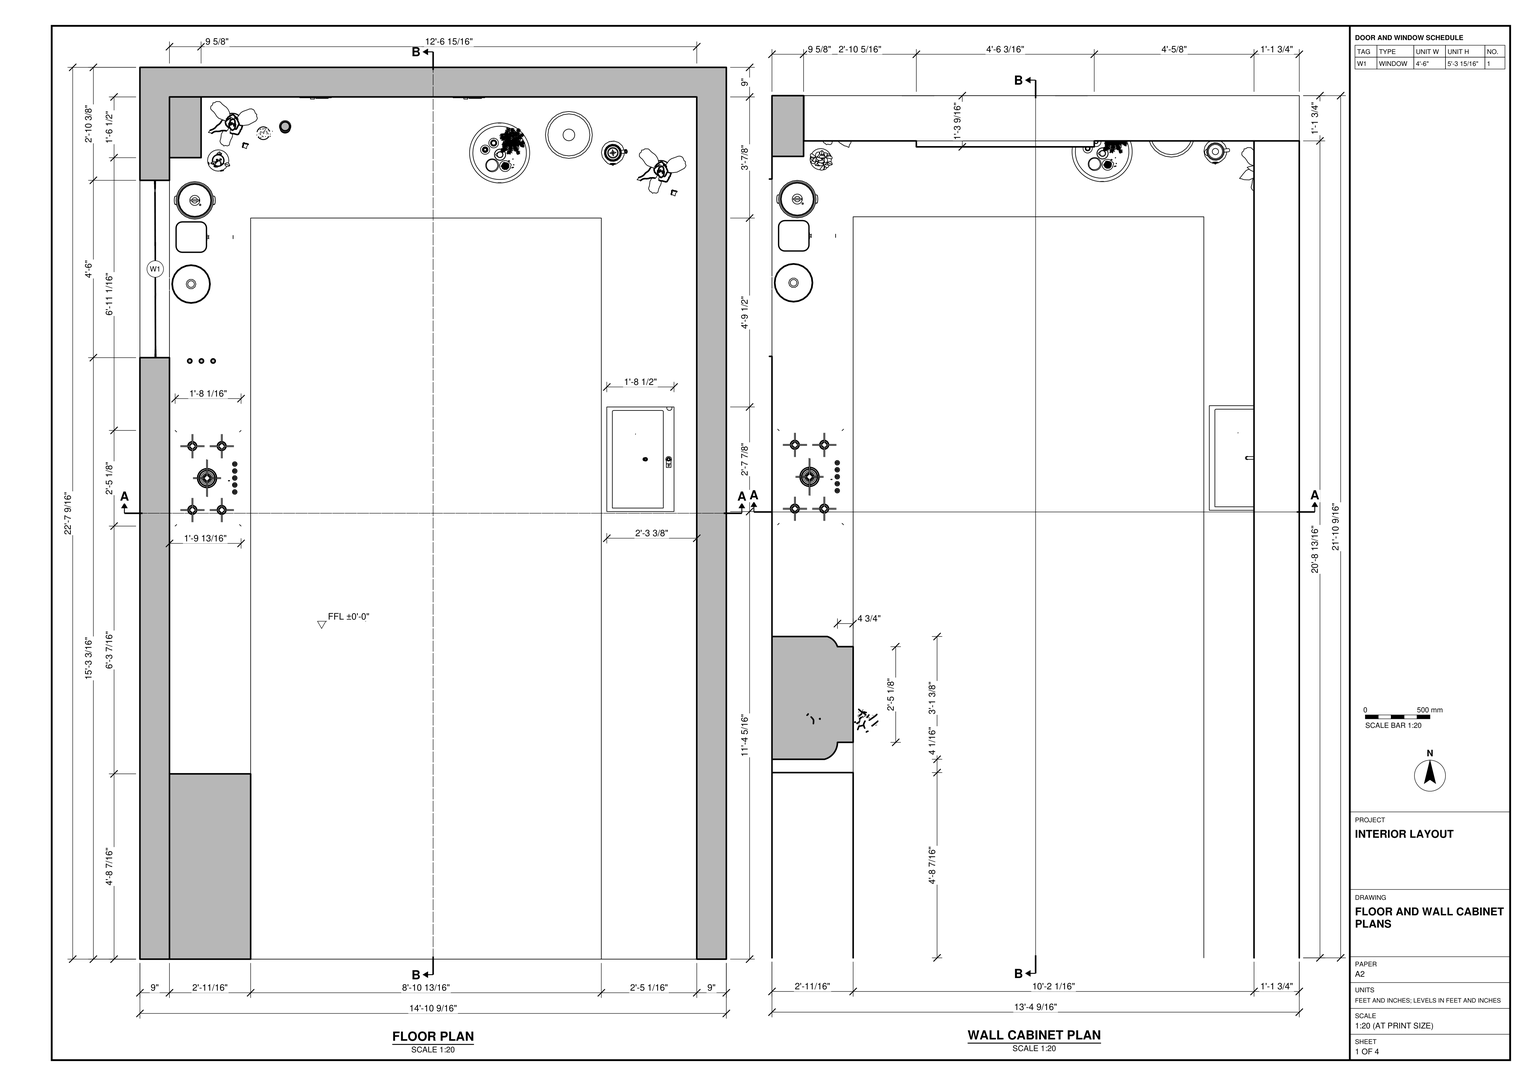
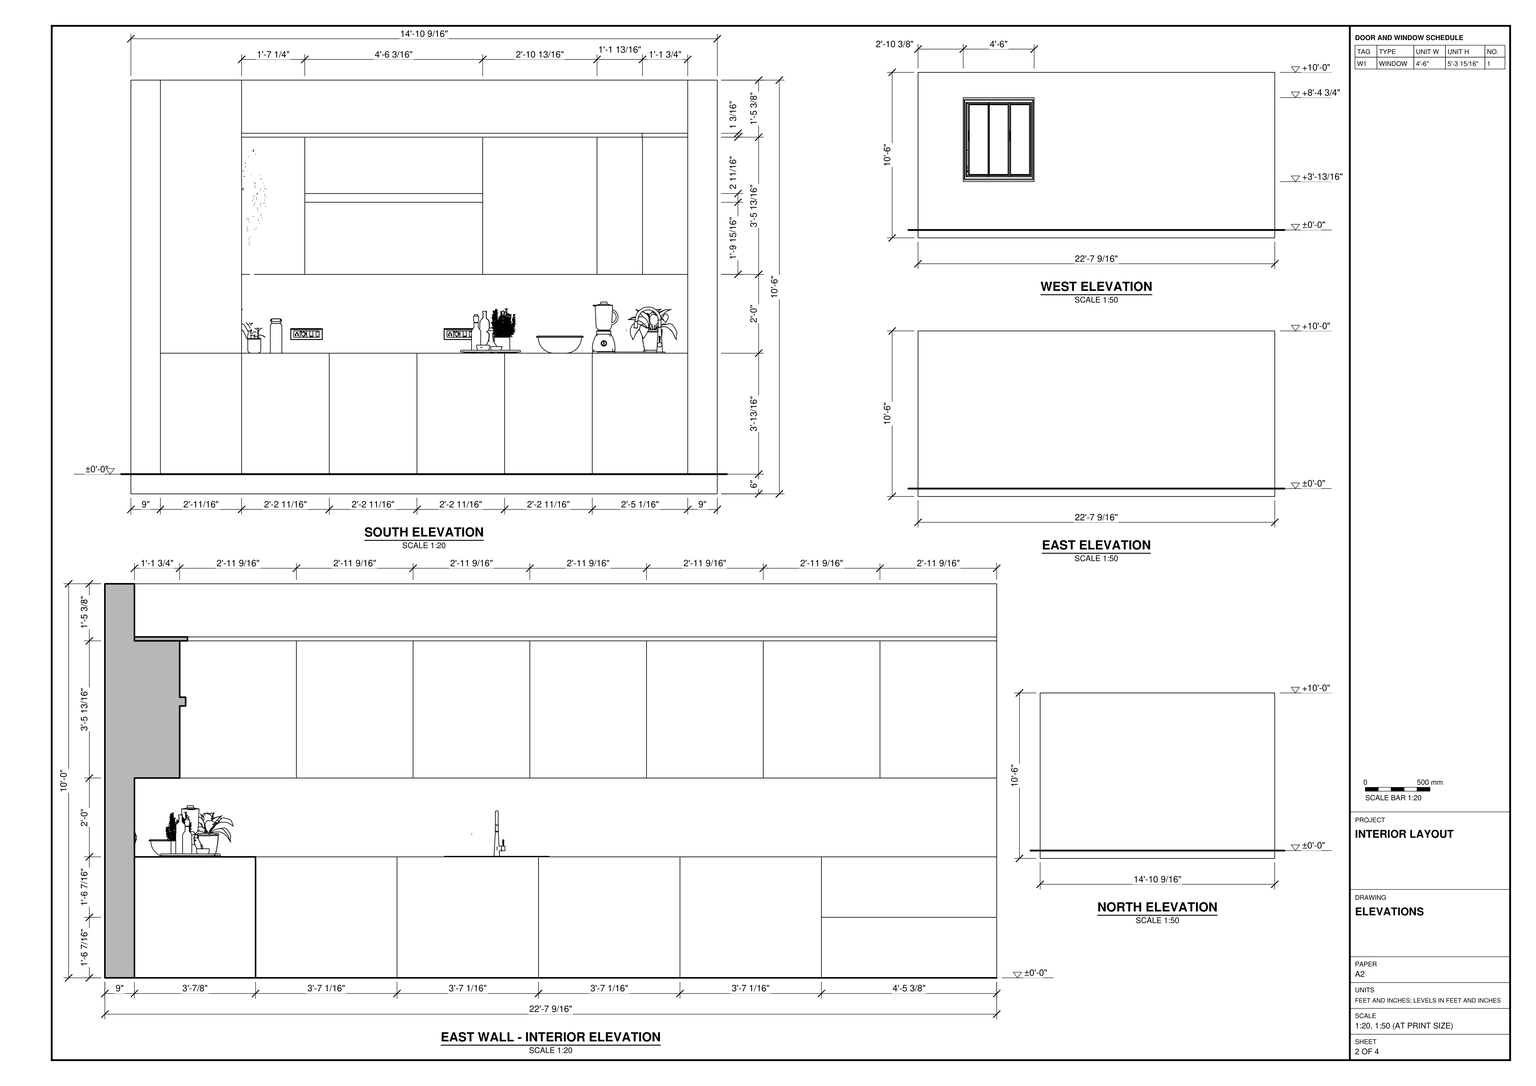
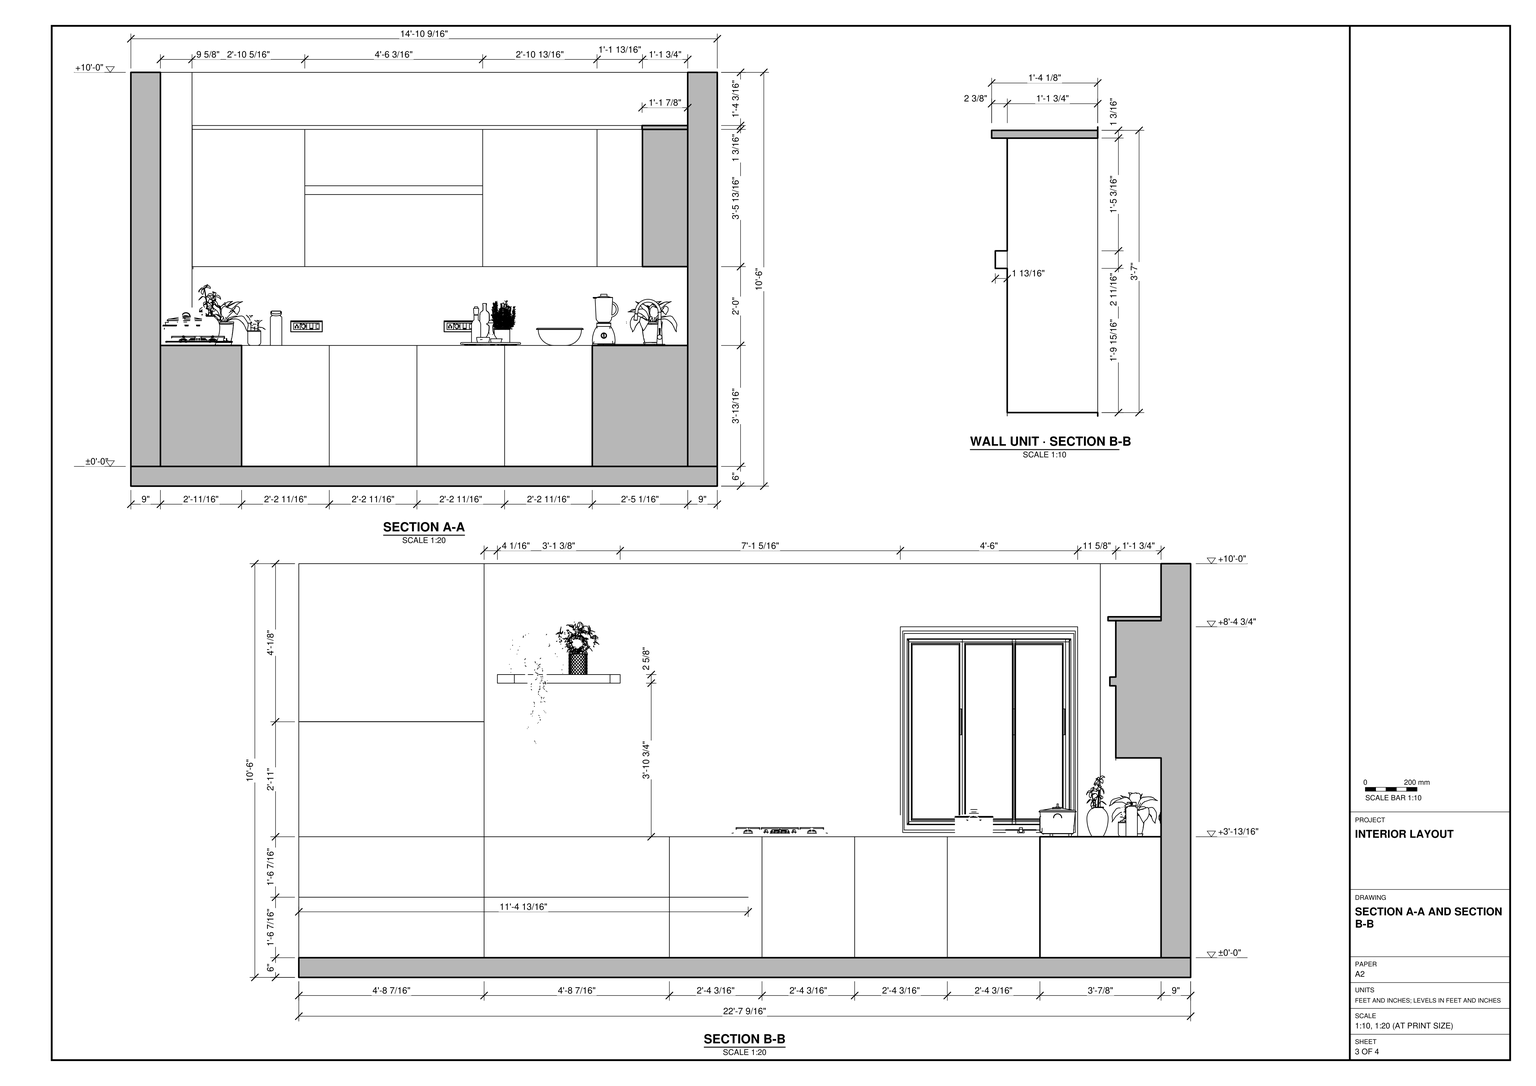
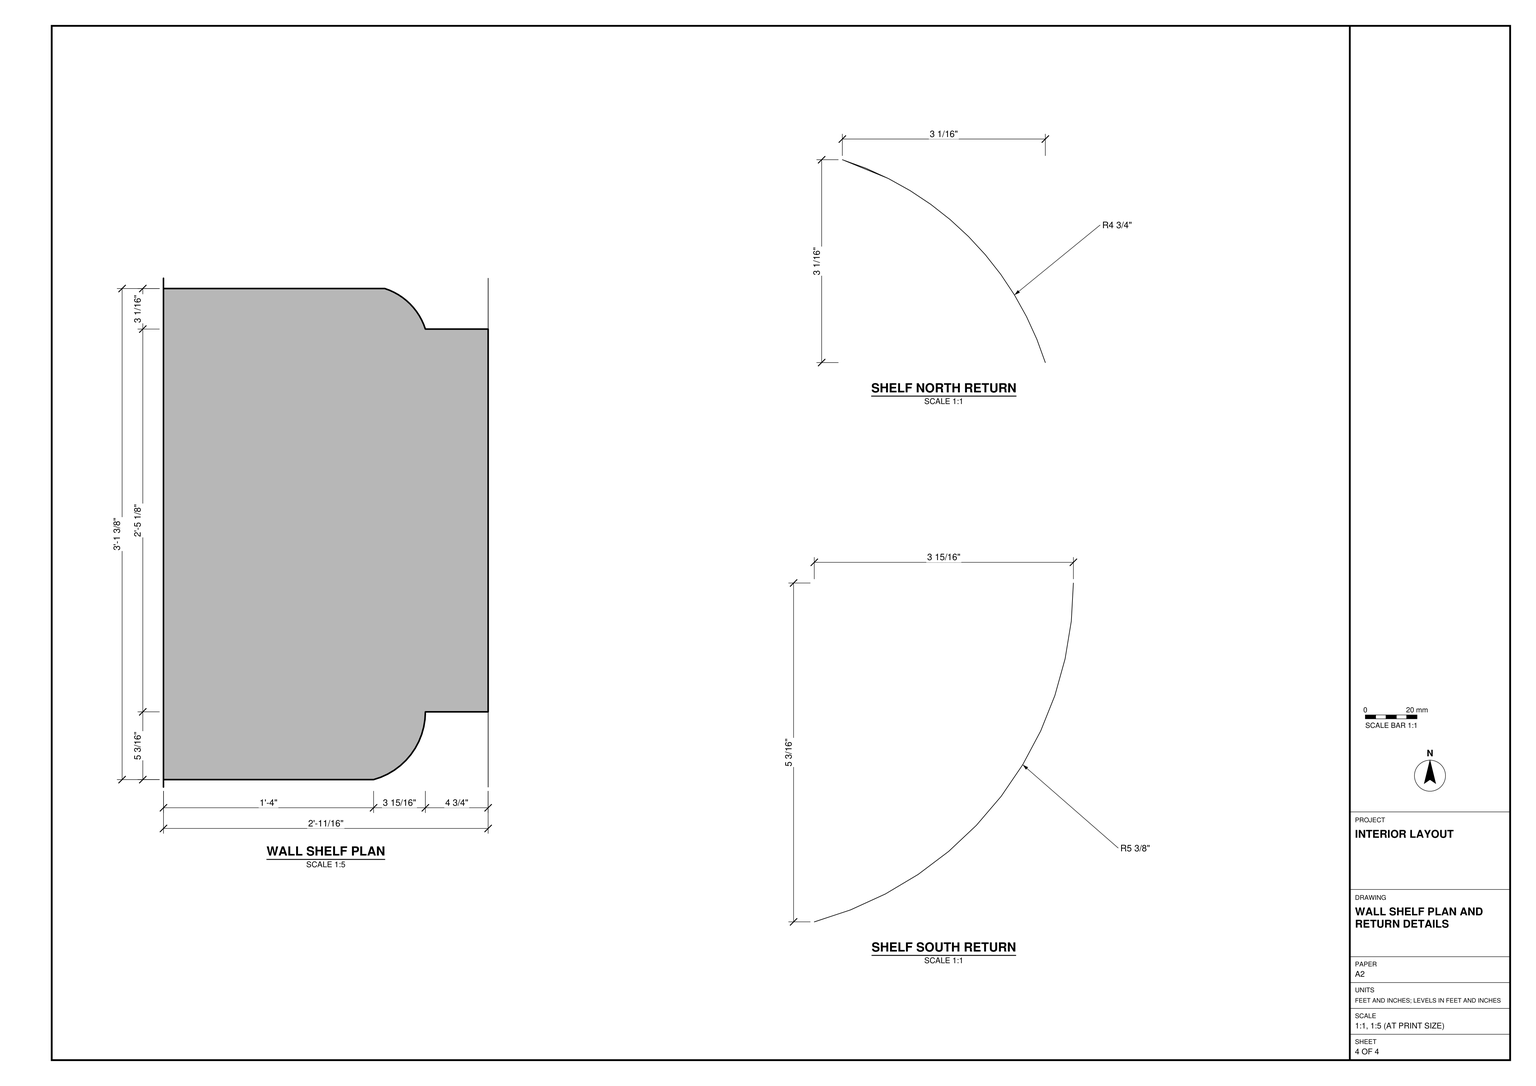
Build the kitchen interior in SketchUp from task_files/diagram_01.pdf. Work in feet and inches. Set the finished floor at ±0'-0". The overall model is 14'-10 9/16" wide, 22'-7 9/16" long and 10'-6" high, including the 6" floor slab below the finished floor. Build the 9" walls on the west, north and east sides, leaving the south end open. Fit the framed window into the west wall at the location and sill height shown.

Run the base cabinets and worktops along both sides and across the north end, keeping the central aisle clear. Place the cooktop on the west run and the sink and tap opposite it on the east run. Use the elevations and sections to set out the cabinet fronts, the tall unit at the open end of the west run and the wall shelf beside it. Model the wall cabinets along the north and east walls, matching their bay widths, projecting top trim and clearance above the worktop. Decor and loose items, including plants, kitchenware and countertop appliances, may be any suitable library components placed as shown.

Keep the shell elements and each piece of joinery or furniture in separate groups or components, and use components for repeated parts. Save one SketchUp model as output_files/open_ended_kitchen_with_u_shaped_cabinetry.skp.

# SketchUp Ruby script. Lengths in inches.
U = 1.inch
M = Sketchup.active_model
def pt(a) = Geom::Point3d.new(a.map { |v| v * U })
def face(e, loops, mat)
  f = e.add_face(loops[0].map { |a| pt(a) })
  loops[1..].each { |l| e.add_face(l.map { |a| pt(a) }).erase! }
  f.material = f.back_material = mat if mat
  f
end
# faces: each face lists its corners as indices into pts; further lists are holes
def faces(e, pts, list, mat = nil) = list.each { |f| face(e, (f[0].is_a?(Array) ? f : [f]).map { |l| l.map { |i| pts[i] } }, mat) }
# xy, xz, yz: faces in a plane at the given z, y or x. An outline is a flat list of corners, or four numbers for a rectangle; further outlines are holes
def ring(l) = l.size == 4 ? [[l[0], l[1]], [l[2], l[1]], [l[2], l[3]], [l[0], l[3]]] : l.each_slice(2).to_a
def flat(e, list, mat, &to3) = list.each { |f| face(e, (f[0].is_a?(Array) ? f : [f]).map { |l| ring(l).map { |u, v| to3.(u, v) } }, mat) }
def xy(e, z, list, mat = nil) = flat(e, list, mat) { |x, y| [x, y, z] }
def xz(e, y, list, mat = nil) = flat(e, list, mat) { |x, z| [x, y, z] }
def yz(e, x, list, mat = nil) = flat(e, list, mat) { |y, z| [x, y, z] }
def lines(e, pts, list) = list.each { |a, b| e.add_line(pt(pts[a]), pt(pts[b])) }
# prism: a flat outline (further loops are holes) pulled along v
def prism(e, loops, v, mat = nil)
  f = face(e, loops, mat); d = Geom::Vector3d.new(v.map { |x| x * U })
  f.pushpull(f.normal.samedirection?(d) ? d.length : -d.length)
end
def box(e, o, s, mat = nil) = prism(e, [[o, [o[0] + s[0], o[1], o[2]], [o[0] + s[0], o[1] + s[1], o[2]], [o[0], o[1] + s[1], o[2]]]], [0, 0, s[2]], mat)
def at(x, y, z, deg = 0) = Geom::Transformation.translation(pt([x, y, z])) * Geom::Transformation.rotation(ORIGIN, Z_AXIS, deg.degrees)
def axes(o, x, y, z) = Geom::Transformation.new([*x, 0, *y, 0, *z, 0, *pt(o).to_a, 1])
def part(name) = M.definitions.add(name)
# library, detail: a bought-in or finely detailed component or shape, given as its bounding box
def library(name, o, s) = part(name).tap { |d| box(d.entities, o, s) }
def detail(e, o, s) = box(e.add_group.entities, o, s)
def put(e, d, t, mat = nil) = e.add_instance(d, t).tap { |i| i.material = mat if mat }
def group(e, t, mat = nil) = e.add_group.tap { |g| g.transformation = t; g.material = mat if mat }.entities
root = M.entities
M.materials.add("[Color M01]").color = [226, 226, 226]
M.materials.add("[Color M04]").color = [142, 142, 142]
M.materials.add("[Tile Border Travertine]").color = [160, 142, 112]
M.materials.add("[Wood Bamboo]").color = [177, 105, 43]
M.materials.add("[Wood Floor Light]").color = [204, 176, 127]
c1 = library("WINDOW",[0,-0.02,0],[73.51,8.29,49.21])
c2 = library("mixer+blender",[-3.57,-3.85,0],[8.2,7.51,15.59])
c3 = library("MixingBowl",[0.58,0.58,0],[14.29,14.29,5.25])
c4 = library("kitchen",[57.57,5.21,10.61],[18.31,18.31,13.72])
c5 = library("Kitchen Pot",[-7.65,-5.94,0],[15.3,11.88,8.57])
c6 = library("Kitchen Pan",[-4.76,-4.76,0],[17.5,9.52,2.79])
c7 = library("Small Plant for Nightstand",[-0.92,-1.74,0],[6.62,5.06,9.81])
c8 = library("Untitled (1)",[45.65,19.99,0],[14.9,14.7,13.43])
c9 = library("Wall switch panel",[0,0,0],[9.65,3.39,0.65])
c10 = library("rice pan",[-4.26,-4.59,0],[12.51,11.42,10.02])
c11 = library("Küche",[96.12,-390.13,36.84],[20.08,114.94,19.93])
c12 = library("sink",[-18.39,0,-25.75],[31.85,20.47,39.62])
c13 = library("water bottle",[-1.75,-2.08,0],[3.5,3.83,10.5])
c14 = library("Untitled\#2",[167.21,48.36,-0.87],[34.16,22.4,50.98])
c15 = library("ARRANJO+ROSAS+BRANCAS",[219.65,-5.05,84.62],[22.21,22.69,31.57])
xy(root,102.625,[[155.67,0,169.5625,246.41],[18.68,246.41,169.5625,262.5625]])
xy(root,103.8125,[[155.67,0,169.5625,0,169.5625,262.5625,18.68,262.5625,18.68,246.41,155.67,246.41]],"[Wood Bamboo]")
xz(root,0,[[155.67,102.625,169.5625,103.8125]],"[Wood Bamboo]")
xz(root,246.41,[[18.68,102.625,155.67,103.8125]],"[Wood Bamboo]")
xz(root,262.5625,[[18.68,102.625,169.5625,103.8125]])
yz(root,18.68,[[246.41,102.625,262.5625,103.8125]])
yz(root,155.67,[[0,102.625,246.41,103.8125]],"[Wood Bamboo]")
yz(root,169.5625,[[0,102.625,246.41,103.8125],[246.41,102.625,262.5625,103.8125]])
p = [[33.72,112.84,18.42],[33.72,136.84,18.42]]
lines(root,p,[[0,1]])
put(root,c1,axes([4.82,183.17,36.84],[-0.0022,0.73462,0],[-0.01952,-0.00006,0],[0,0,1.29921]))
put(root,c2,at(144.01,245.47,36.84))
put(root,c3,at(122.9,243.27,36.84))
put(root,c4,at(42.8,231.15,26.23))
put(root,c5,at(15.57,205.57,36.84))
put(root,c6,at(15.64,219.88,36.84))
put(root,c7,at(35.31,250.67,36.84))
put(root,c8,at(-24.8,226.8,36.84))
put(root,c9,axes([95.35,262.54,40.97],[1,0,0],[0,0,1],[0,-1,0]))
put(root,c9,axes([48.67,262.54,40.97],[1,0,0],[0,0,1],[0,-1,0]))
put(root,c10,at(14.71,229.9375,36.84))
put(root,c11,at(-85.4,522,0))
put(root,c12,at(142.17,149.76,37.03,-90))
put(root,c8,at(105.72,212.41,36.84))
put(root,c13,at(44.22,253.6,36.84))
put(root,c14,at(-151.33,13.47,53.1))
put(root,c15,axes([-210.01,80.1875,34.69],[1,0,0],[0,0.72365,0],[0,0,0.59]))
g1 = group(root,at(0,82.5625,0),"[Color M01]")
xy(g1,0,[[0,-82.5625,0,189,178.5625,189,178.5625,-82.5625,169.5625,-82.5625,169.5625,180,9,180,9,-82.5625]],"[Color M01]")
xy(g1,36.84,[[0,100.6,9,154.6],[9,161.5,18.625,180]],"[Color M01]")
xy(g1,60.84,[[155.78,-82.5625,169.5625,166.22],[18.68,166.22,169.5625,180]],"[Color M01]")
xy(g1,82.79,[[52.96,164.41,107.13,166.22]],"[Color M01]")
xy(g1,85.46,[[52.96,164.41,107.13,166.22]],"[Color M01]")
xy(g1,100.78,[[0,100.6,9,154.6]],"[Color M01]")
xy(g1,102.625,[[155.78,-82.5625,169.5625,166.22],[18.68,166.22,169.5625,180]],"[Color M01]")
xy(g1,120,[[0,-82.5625,9,-82.5625,9,180,169.5625,180,169.5625,-82.5625,178.5625,-82.5625,178.5625,189,0,189]],"[Color M01]")
xy(g1,120,[[9,161.5,18.625,180]],"[Wood Bamboo]")
xz(g1,-82.5625,[[0,0,9,120],[169.5625,0,178.5625,120],[155.78,60.84,169.5625,102.625]],"[Color M01]")
xz(g1,100.6,[[0,36.84,9,100.78]],"[Color M01]")
xz(g1,154.6,[[0,36.84,9,100.78]],"[Color M04]")
xz(g1,161.5,[[9,36.84,18.625,120]],"[Wood Bamboo]")
xz(g1,164.41,[[52.96,82.79,107.13,85.46]],"[Color M01]")
xz(g1,166.22,[[18.68,60.84,52.96,102.625],[52.96,60.84,107.13,82.79],[107.13,60.84,141.95,102.625],[141.95,60.84,155.78,102.625],[155.78,60.84,169.5625,102.625],
  [52.96,85.46,107.13,102.625]],"[Color M01]")
xz(g1,180,[[9,36.84,18.625,60.84],[9,60.84,18.625,102.625],[9,102.625,18.625,120]],"[Color M01]")
xz(g1,180,[[18.625,102.625,169.5625,120]],"[Color M04]")
xz(g1,189,[[0,0,178.5625,120]],"[Color M01]")
yz(g1,0,[[[-82.5625,0,189,120],[100.6,36.84,154.6,100.78]]],"[Color M01]")
yz(g1,9,[[[-82.5625,0,180,0,180,36.84,161.5,36.84,161.5,120,-82.5625,120],[100.6,36.84,154.6,100.78]],[161.5,36.84,180,60.84],[161.5,60.84,180,102.625],[161.5,102.625,180,120]],"[Color M01]")
yz(g1,18.625,[[161.5,36.84,180,120]],"[Wood Bamboo]")
yz(g1,18.68,[[166.22,60.84,180,102.625]],"[Color M01]")
yz(g1,52.96,[[164.41,82.79,166.22,85.46]],"[Color M01]")
yz(g1,107.13,[[164.41,82.79,166.22,85.46]],"[Color M01]")
yz(g1,155.78,[[-82.5625,60.84,-47.02,102.625],[-47.02,60.84,-11.48,102.625],[-11.48,60.84,24.06,102.625],[24.06,60.84,59.6,102.625],[59.6,60.84,95.14,102.625],
  [95.14,60.84,130.68,102.625],[130.68,60.84,166.22,102.625]],"[Color M01]")
yz(g1,169.5625,[[-82.5625,60.84,166.22,102.625]],"[Color M01]")
yz(g1,169.5625,[[-82.5625,0,180,60.84],[-82.5625,102.625,180,120]],"[Color M04]")
yz(g1,178.5625,[[-82.5625,0,189,120]],"[Color M01]")
p = [[140.5,-29.2,18.42],[140.5,-82.5625,18.42],[33.72,-82.5625,18.42],[33.72,-26.14,18.42],[33.72,30.28,18.42],[18.92,166.22,60.84],
  [18.92,166.22,60.125],[33.72,-82.5625,71.85],[33.72,-26.14,71.85]]
lines(g1,p,[[0,1],[2,3],[3,4],[5,6],[7,8]])
g2 = group(g1,at(9,-82.5625,0),"[Color M01]")
xy(g2,0,[[0,0,0,262.5625,160.5625,262.5625,160.5625,0,131.5,0,131.5,225.68,24.72,225.68,24.72,0]])
xy(g2,36.84,[[0,0,24.72,0,24.72,225.68,131.5,225.68,131.5,0,160.5625,0,160.5625,262.5625,0,262.5625]])
xz(g2,0,[[131.5,0,160.5625,36.84]])
xz(g2,0,[[0,0,24.72,36.84]],"[Wood Bamboo]")
xz(g2,225.68,[[24.72,0,51.41,36.84],[51.41,0,78.11,36.84],[78.11,0,104.8,36.84],[104.8,0,131.5,36.84]])
xz(g2,262.5625,[[0,0,160.5625,36.84]])
yz(g2,0,[[0,0,262.5625,36.84]])
yz(g2,24.72,[[56.42,0,112.84,18.42],[112.84,0,141.05,36.84],[141.05,0,169.26,36.84],[169.26,0,197.47,36.84],[197.47,0,225.68,36.84]])
yz(g2,24.72,[[0,0,56.42,36.84],[56.42,18.42,112.84,36.84]],"[Wood Bamboo]")
yz(g2,131.5,[[53.36,0,96.44,36.84],[96.44,0,139.52,36.84],[139.52,0,182.6,36.84],[182.6,0,225.68,36.84]])
yz(g2,131.5,[[0,0,53.36,36.84]],"[Wood Bamboo]")
yz(g2,160.5625,[[0,0,262.5625,36.84]])
p = [[160.5625,262.5625,60.84],[0,262.5625,60.84]]
lines(g2,p,[[0,1]])
g3 = group(g1,at(9,-82.5625,36.84),"[Wood Bamboo]")
xy(g3,0,[[0,0,24.72,56.42]])
xy(g3,83.16,[[0,0,24.72,56.42]])
xz(g3,0,[[0,0,24.72,83.16]])
xz(g3,56.42,[[0,0,24.72,83.16]])
yz(g3,0,[[0,0,56.42,83.16]])
yz(g3,24.72,[[0,0,56.42,35.06]])
yz(g3,24.72,[[0,35.06,56.42,83.16]],"[Wood Bamboo]")
g4 = group(g1,at(9,-26.14,83.6),"[Wood Floor Light]")
xy(g4,0,[[0,4.05,0,41.4375,16.85,41.4375,17.2,41.31,17.55,41.15,17.88,40.97,18.19,40.76,18.49,40.52,18.77,40.27,19.02,39.99,19.26,39.69,19.47,39.38,19.65,39.05,19.81,38.7,19.9375,38.35,24.72,38.35,24.72,9.21,19.9375,9.21,19.91,8.63,19.8125,8.06,19.66,7.5,19.4375,6.96,19.17,6.44,18.84,5.96,18.46,5.52,18.04,5.12,17.57,4.77,17.07,4.47,16.55,4.23,15.99,4.05]])
xy(g4,2.625,[[0,4.05,15.99,4.05,16.55,4.23,17.07,4.47,17.57,4.77,18.04,5.12,18.46,5.52,18.84,5.96,19.17,6.44,19.4375,6.96,19.66,7.5,19.8125,8.06,19.91,8.63,19.9375,9.21,24.72,9.21,24.72,38.35,19.9375,38.35,19.81,38.7,19.65,39.05,19.47,39.38,19.26,39.69,19.02,39.99,18.77,40.27,18.49,40.52,18.19,40.76,17.88,40.97,17.55,41.15,17.2,41.31,16.85,41.4375,0,41.4375]],"[Wood Floor Light]")
xz(g4,4.05,[[0,0,15.99,2.625]])
xz(g4,9.21,[[19.9375,0,24.72,2.625]])
xz(g4,38.35,[[19.9375,0,24.72,2.625]])
xz(g4,41.4375,[[0,0,16.85,2.625]])
yz(g4,0,[[4.05,0,41.4375,2.625]])
yz(g4,24.72,[[9.21,0,38.35,2.625]],"[Wood Floor Light]")
p = [[16.55,4.23,2.625],[15.99,4.05,2.625],[15.99,4.05,0],[16.55,4.23,0],[17.07,4.47,2.625],[17.07,4.47,0],
  [17.57,4.77,2.625],[17.57,4.77,0],[18.04,5.12,2.625],[18.04,5.12,0],[18.46,5.52,2.625],[18.46,5.52,0],
  [18.84,5.96,2.625],[18.84,5.96,0],[19.17,6.44,2.625],[19.17,6.44,0],[19.4375,6.96,2.625],[19.4375,6.96,0],
  [19.66,7.5,2.625],[19.66,7.5,0],[19.8125,8.06,2.625],[19.8125,8.06,0],[19.91,8.63,2.625],[19.91,8.63,0],
  [19.9375,9.21,2.625],[19.9375,9.21,0],[19.81,38.7,2.625],[19.9375,38.35,2.625],[19.9375,38.35,0],[19.81,38.7,0],
  [19.65,39.05,2.625],[19.65,39.05,0],[19.47,39.38,2.625],[19.47,39.38,0],[19.26,39.69,2.625],[19.26,39.69,0],
  [19.02,39.99,2.625],[19.02,39.99,0],[18.77,40.27,2.625],[18.77,40.27,0],[18.49,40.52,2.625],[18.49,40.52,0],
  [18.19,40.76,2.625],[18.19,40.76,0],[17.88,40.97,2.625],[17.88,40.97,0],[17.55,41.15,2.625],[17.55,41.15,0],
  [17.2,41.31,2.625],[17.2,41.31,0],[16.85,41.4375,2.625],[16.85,41.4375,0],[0,0,0],[0,0,2.625]]
faces(g4,p,[[0,1,2,3],[4,0,3,5],[6,4,5,7],[8,6,7,9],[10,8,9,11],[12,10,11,13],[14,12,13,15],[16,14,15,17],
  [18,16,17,19],[20,18,19,21],[22,20,21,23],[24,22,23,25],[26,27,28,29],[30,26,29,31],[32,30,31,33],[34,32,33,35],
  [36,34,35,37],[38,36,37,39],[40,38,39,41],[42,40,41,43],[44,42,43,45],[46,44,45,47],[48,46,47,49],[50,48,49,51]],"[Wood Floor Light]")
lines(g4,p,[[52,53]])
g5 = group(g1,at(9,180,0),"[Color M04]")
xz(g5,0,[[0,0,160.5625,0,160.5625,60.84,9.625,60.84,9.625,36.84,0,36.84]],"[Color M04]")
g6 = group(root,at(0,0,120))
xy(g6,-126,[[0,0,178.5625,271.5625]])
xy(g6,-120,[[0,0,178.5625,271.5625]],"[Tile Border Travertine]")
xz(g6,0,[[0,-126,178.5625,-120]])
xz(g6,271.5625,[[0,-126,178.5625,-120]])
yz(g6,0,[[0,-126,271.5625,-120]])
yz(g6,178.5625,[[0,-126,271.5625,-120]])
